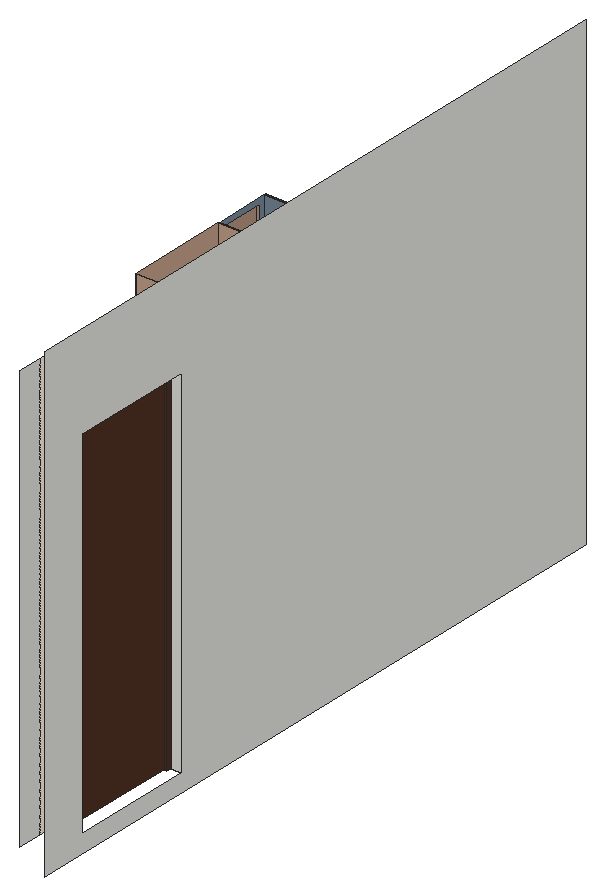
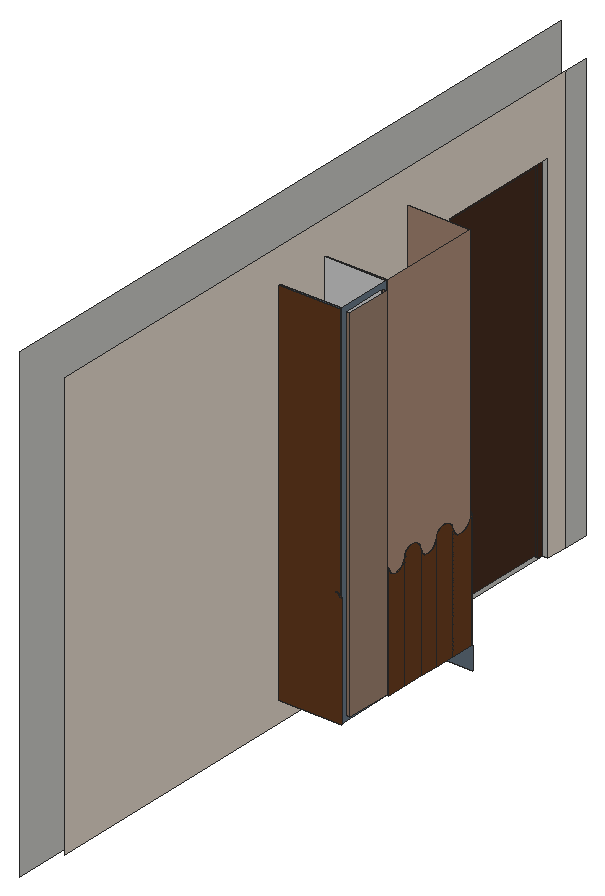
# SketchUp Ruby script. Lengths in inches.
U = 1.inch
M = Sketchup.active_model
def pt(a) = Geom::Point3d.new(a.map { |v| v * U })
def face(e, loops, mat)
  f = e.add_face(loops[0].map { |a| pt(a) })
  loops[1..].each { |l| e.add_face(l.map { |a| pt(a) }).erase! }
  f.material = f.back_material = mat if mat
  f
end
# faces: each face lists its corners as indices into pts; further lists are holes
def faces(e, pts, list, mat = nil) = list.each { |f| face(e, (f[0].is_a?(Array) ? f : [f]).map { |l| l.map { |i| pts[i] } }, mat) }
# xy, xz, yz: faces in a plane at the given z, y or x. An outline is a flat list of corners, or four numbers for a rectangle; further outlines are holes
def ring(l) = l.size == 4 ? [[l[0], l[1]], [l[2], l[1]], [l[2], l[3]], [l[0], l[3]]] : l.each_slice(2).to_a
def flat(e, list, mat, &to3) = list.each { |f| face(e, (f[0].is_a?(Array) ? f : [f]).map { |l| ring(l).map { |u, v| to3.(u, v) } }, mat) }
def xy(e, z, list, mat = nil) = flat(e, list, mat) { |x, y| [x, y, z] }
def xz(e, y, list, mat = nil) = flat(e, list, mat) { |x, z| [x, y, z] }
def yz(e, x, list, mat = nil) = flat(e, list, mat) { |y, z| [x, y, z] }
def lines(e, pts, list) = list.each { |a, b| e.add_line(pt(pts[a]), pt(pts[b])) }
# prism: a flat outline (further loops are holes) pulled along v
def prism(e, loops, v, mat = nil)
  f = face(e, loops, mat); d = Geom::Vector3d.new(v.map { |x| x * U })
  f.pushpull(f.normal.samedirection?(d) ? d.length : -d.length)
end
def box(e, o, s, mat = nil) = prism(e, [[o, [o[0] + s[0], o[1], o[2]], [o[0] + s[0], o[1] + s[1], o[2]], [o[0], o[1] + s[1], o[2]]]], [0, 0, s[2]], mat)
def at(x, y, z, deg = 0) = Geom::Transformation.translation(pt([x, y, z])) * Geom::Transformation.rotation(ORIGIN, Z_AXIS, deg.degrees)
def axes(o, x, y, z) = Geom::Transformation.new([*x, 0, *y, 0, *z, 0, *pt(o).to_a, 1])
def part(name) = M.definitions.add(name)
# library, detail: a bought-in or finely detailed component or shape, given as its bounding box
def library(name, o, s) = part(name).tap { |d| box(d.entities, o, s) }
def detail(e, o, s) = box(e.add_group.entities, o, s)
def put(e, d, t, mat = nil) = e.add_instance(d, t).tap { |i| i.material = mat if mat }
def group(e, t, mat = nil) = e.add_group.tap { |g| g.transformation = t; g.material = mat if mat }.entities
root = M.entities
M.materials.add("Polis06_194").color = [79, 50, 36]
M.materials.add("[0009_Linen]").color = [197, 160, 138]
M.materials.add("[0110_LightSlateGray]1").color = [119, 136, 153]
M.materials.add("[0111_SlateGray]").color = [255, 255, 255]
M.materials.add("[Color D01]").color = [255, 242, 228]
M.materials.add("[Fencing Lattice Natural]").color = [179, 148, 127]
M.materials.add("[Wood Veneer 01]").color = [120, 70, 37]
c1 = part("Flush door")
xy(c1.entities,0,[[0,0,4.72,1.18],[0,34.25,4.72,35.43]],"Polis06_194")
xy(c1.entities,85.26,[[0,1.18,4.72,34.25]],"Polis06_194")
xy(c1.entities,86.61,[[0,0,4.72,35.43]],"Polis06_194")
xz(c1.entities,0,[[0,0,4.72,86.61]],"Polis06_194")
xz(c1.entities,1.18,[[0,0,2.36,85.26],[2.36,0,4.72,85.26]],"Polis06_194")
xz(c1.entities,34.25,[[0,0,4.72,85.26]],"Polis06_194")
xz(c1.entities,35.43,[[0,0,4.72,86.61]],"Polis06_194")
yz(c1.entities,0,[[0,0,1.18,86.61],[34.25,0,35.43,86.61],[1.18,85.26,34.25,86.61]],"Polis06_194")
yz(c1.entities,2.36,[[1.18,0,34.25,0,34.25,85.21,1.18,85.26]],"Polis06_194")
yz(c1.entities,4.72,[[0,0,1.18,86.61],[34.25,0,35.43,86.61],[1.18,85.26,34.25,86.61]],"Polis06_194")
c2 = library("Spot Light\#1",[-5.1,-5.1,-11.05],[10.2,10.2,11.05])
xy(root,13.75,[[535.73,77.57,535.73,78.14,540.39,78.14,539.85,77.57],[539.85,77.57,540.39,78.14,544.32,78.14,543.91,77.57],[543.91,77.57,544.32,78.14,549.07,78.14,548.8,77.57],[548.8,77.57,549.07,78.14,553.89,78.14,553.76,77.57],[553.76,77.57,553.89,78.14,558.07,78.14,558.07,77.57]],"[0009_Linen]")
xy(root,15.58,[[536.14,116.57,553.2,132.48]],"[0110_LightSlateGray]1")
xy(root,15.58,[[534.57,116.57,536.14,132.48]],"[Fencing Lattice Natural]")
xy(root,34.7,[[536.14,116.57,553.2,132.48]],"[0110_LightSlateGray]1")
xy(root,36.7,[[536.14,116.57,553.2,132.48]],"[0110_LightSlateGray]1")
xy(root,55.82,[[536.14,116.57,553.2,132.48]],"[0110_LightSlateGray]1")
xz(root,16.33,[[558.07,6.125,566.72,131.66]])
xz(root,59.9,[[558.07,6.125,566.72,131.66]])
xz(root,77.57,[[535.73,13.75,539.85,13.75,539.85,53.75,539.84,54.31,539.67,54.85,539.34,55.32,538.9,55.6875,538.37,55.92,537.79,56,537.22,55.92,536.6875,55.6875,536.24,55.32,535.92,54.85,535.75,54.31,535.73,53.75],[539.85,13.75,543.91,13.75,543.91,53.75,543.84,53.24,543.64,52.77,543.32,52.36,542.9,52.05,542.41,51.85,541.88,51.78,541.36,51.85,540.87,52.05,540.45,52.36,540.125,52.77,539.92,53.24,539.85,53.75],[543.91,13.75,548.8,13.75,548.8,53.75,548.73,54.375,548.5,54.96,548.11,55.47,547.6,55.86,547,56.1,546.36,56.1875,545.71,56.1,545.11,55.86,544.6,55.47,544.22,54.96,543.98,54.375,543.91,53.75],[548.8,13.75,553.76,13.75,553.76,53.75,553.61,53.18,553.33,52.67,552.93,52.23,552.4375,51.9,551.88,51.7,551.28,51.625,550.68,51.7,550.12,51.9,549.63,52.23,549.23,52.67,548.95,53.18,548.8,53.75],[553.76,13.75,558.07,13.75,558.07,53.75,558.0625,54.34,557.88,54.91,557.55,55.41,557.08,55.8,556.52,56.04,555.92,56.125,555.31,56.04,554.75,55.8,554.29,55.41,553.95,54.91,553.77,54.34,553.76,53.75]],"[Wood Veneer 01]")
xz(root,78.14,[[536.14,13.75,536.14,53.75,535.73,53.75,535.75,54.31,535.92,54.85,536.14,55.16,536.24,55.32,536.6875,55.6875,537.22,55.92,537.79,56,538.37,55.92,538.9,55.6875,539.34,55.32,539.67,54.85,539.84,54.31,539.85,53.75,539.92,53.24,540.125,52.77,540.45,52.36,540.87,52.05,541.36,51.85,541.88,51.78,542.41,51.85,542.9,52.05,543.32,52.36,543.64,52.77,543.84,53.24,543.91,53.75,543.98,54.375,544.22,54.96,544.6,55.47,545.11,55.86,545.71,56.1,546.36,56.1875,547,56.1,547.6,55.86,548.11,55.47,548.5,54.96,548.73,54.375,548.8,53.75,548.95,53.18,549.23,52.67,549.63,52.23,550.12,51.9,550.68,51.7,551.28,51.625,551.88,51.7,552.4375,51.9,552.93,52.23,553.33,52.67,553.61,53.18,553.76,53.75,553.77,54.34,553.95,54.91,554.29,55.41,554.75,55.8,555.31,56.04,555.92,56.125,556.52,56.04,557.08,55.8,557.55,55.41,557.88,54.91,558.0625,54.34,558.07,53.75,558.07,144.125,536.14,144.125,536.14,55.16,536.24,55.32,536.6875,55.6875,537.22,55.92,537.79,56,538.37,55.92,538.9,55.6875,539.34,55.32,539.67,54.85,539.84,54.31,539.85,53.75,539.92,53.24,540.125,52.77,540.45,52.36,540.87,52.05,541.36,51.85,541.88,51.78,542.41,51.85,542.9,52.05,543.32,52.36,543.64,52.77,543.84,53.24,543.91,53.75,543.98,54.375,544.22,54.96,544.6,55.47,545.11,55.86,545.71,56.1,546.36,56.1875,547,56.1,547.6,55.86,548.11,55.47,548.5,54.96,548.73,54.375,548.8,53.75,548.95,53.18,549.23,52.67,549.63,52.23,550.12,51.9,550.68,51.7,551.28,51.625,551.88,51.7,552.4375,51.9,552.93,52.23,553.33,52.67,553.61,53.18,553.76,53.75,553.77,54.34,553.95,54.91,554.29,55.41,554.75,55.8,555.31,56.04,555.92,56.125,556.52,56.04,557.08,55.8,557.55,55.41,557.88,54.91,558.0625,54.34,558.07,53.75,558.07,13.75],[536.14,13.75,558.07,13.75,558.07,53.75,558.0625,54.34,557.88,54.91,557.55,55.41,557.08,55.8,556.52,56.04,555.92,56.125,555.31,56.04,554.75,55.8,554.29,55.41,553.95,54.91,553.77,54.34,553.76,53.75,553.61,53.18,553.33,52.67,552.93,52.23,552.4375,51.9,551.88,51.7,551.28,51.625,550.68,51.7,550.12,51.9,549.63,52.23,549.23,52.67,548.95,53.18,548.8,53.75,548.73,54.375,548.5,54.96,548.11,55.47,547.6,55.86,547,56.1,546.36,56.1875,545.71,56.1,545.11,55.86,544.6,55.47,544.22,54.96,543.98,54.375,543.91,53.75,543.84,53.24,543.64,52.77,543.32,52.36,542.9,52.05,542.41,51.85,541.88,51.78,541.36,51.85,540.87,52.05,540.45,52.36,540.125,52.77,539.92,53.24,539.85,53.75,539.84,54.31,539.67,54.85,539.34,55.32,538.9,55.6875,538.37,55.92,537.79,56,537.22,55.92,536.6875,55.6875,536.24,55.32,536.14,55.16]],"[0009_Linen]")
xz(root,78.14,[[535.07,6.125,558.07,13.75]],"[0110_LightSlateGray]1")
xz(root,78.14,[[535.64,13.75,535.73,53.75],[535.73,13.75,536.14,53.75]],"[Wood Veneer 01]")
xz(root,114.14,[[535.64,13.75,535.64,53.75,536.14,53.75,536.14,144.125,558.07,144.125,558.07,13.75]],"[0009_Linen]")
xz(root,114.74,[[536.14,13.75,558.07,144.125]],"[0111_SlateGray]")
xz(root,116.57,[[536.14,34.7,553.2,36.7],[536.14,55.82,553.2,57.82]])
xz(root,116.57,[[536.14,15.58,553.2,34.7],[536.14,36.7,553.2,55.82]],"[0110_LightSlateGray]1")
xz(root,116.57,[[534.57,15.58,536.14,142.3]],"[Fencing Lattice Natural]")
xz(root,132.48,[[536.14,15.58,553.2,34.7],[536.14,36.7,553.2,55.82]],"[0110_LightSlateGray]1")
xz(root,132.48,[[534.57,15.58,536.14,142.3]],"[Fencing Lattice Natural]")
xz(root,134.3125,[[536.14,13.75,558.07,144.125]],"[0110_LightSlateGray]1")
xz(root,134.91,[[535.64,13.75,558.07,13.75,558.07,144.125,536.14,144.125,536.14,53.75,535.64,53.75]],"[Wood Veneer 01]")
yz(root,534.57,[[116.57,15.58,132.48,142.3]],"[Fencing Lattice Natural]")
yz(root,535.64,[[78.14,13.75,78.14,53.75,78.48,52.93,78.98,52.19,79.64,51.58,80.4,51.13,81.25,50.85,82.14,50.75,83.02,50.85,83.87,51.13,84.64,51.58,85.29,52.19,85.8,52.93,86.14,53.75,86.14,13.75],[86.14,13.75,86.14,53.75,86.36,54.55,86.77,55.28,87.33,55.9,88.03,56.36,88.81,56.65,89.64,56.75,90.47,56.65,91.25,56.36,91.94,55.9,92.51,55.28,92.91,54.55,93.14,53.75,93.14,13.75],[93.14,13.75,93.14,53.75,93.36,52.95,93.77,52.22,94.33,51.6,95.03,51.14,95.81,50.85,96.64,50.75,97.47,50.85,98.25,51.14,98.94,51.6,99.51,52.22,99.91,52.95,100.14,53.75,100.14,13.75],[100.14,13.75,100.14,53.75,100.36,54.55,100.77,55.28,101.33,55.9,102.03,56.36,102.81,56.65,103.64,56.75,104.47,56.65,105.25,56.36,105.94,55.9,106.51,55.28,106.91,54.55,107.14,53.75,107.14,13.75],[107.14,13.75,107.14,53.75,107.36,52.95,107.77,52.22,108.33,51.6,109.03,51.14,109.81,50.85,110.64,50.75,111.47,50.85,112.25,51.14,112.94,51.6,113.51,52.22,113.91,52.95,114.14,53.75,114.14,13.75]],"[Wood Veneer 01]")
yz(root,535.73,[[77.57,13.75,78.14,53.75]],"[Wood Veneer 01]")
yz(root,536.14,[[82.14,50.75,81.25,50.85,80.4,51.13,79.64,51.58,78.98,52.19,78.48,52.93,78.14,53.75,78.14,144.125,114.14,144.125,114.14,53.75,113.91,52.95,113.51,52.22,112.94,51.6,112.25,51.14,111.47,50.85,110.64,50.75,109.81,50.85,109.03,51.14,108.33,51.6,107.77,52.22,107.36,52.95,107.14,53.75,106.91,54.55,106.51,55.28,105.94,55.9,105.25,56.36,104.47,56.65,103.64,56.75,102.81,56.65,102.03,56.36,101.33,55.9,100.77,55.28,100.36,54.55,100.14,53.75,99.91,52.95,99.51,52.22,98.94,51.6,98.25,51.14,97.47,50.85,96.64,50.75,95.81,50.85,95.03,51.14,94.33,51.6,93.77,52.22,93.36,52.95,93.14,53.75,92.91,54.55,92.51,55.28,91.94,55.9,91.25,56.36,90.47,56.65,89.64,56.75,88.81,56.65,88.03,56.36,87.33,55.9,86.77,55.28,86.36,54.55,86.14,53.75,85.8,52.93,85.29,52.19,84.64,51.58,83.87,51.13,83.02,50.85]],"[0009_Linen]")
yz(root,536.14,[[[114.74,13.75,134.3125,144.125],[116.57,15.58,132.48,142.3]],[116.57,34.7,132.48,36.7],[116.57,55.82,132.48,57.82]],"[0110_LightSlateGray]1")
yz(root,553.2,[[116.57,15.58,132.48,34.7],[116.57,36.7,132.48,55.82]],"[0110_LightSlateGray]1")
yz(root,558.07,[[0,6.125,8.65,155.75]])
yz(root,558.07,[[77.57,13.75,78.14,53.75]],"[0009_Linen]")
yz(root,558.07,[[8.65,6.125,8.65,155.75,228.1,155.75,228.1,6.125,59.9,6.125,59.9,131.66,16.33,131.66,16.33,6.125]],"[Color D01]")
yz(root,566.72,[[[0,0,236.75,164.75],[16.33,6.125,59.9,131.66]]])
p = [[536.14,80.4,51.13],[536.14,81.25,50.85],[535.64,81.25,50.85],[535.64,80.4,51.13],[536.14,82.14,50.75],[535.64,82.14,50.75],
  [536.14,83.02,50.85],[535.64,83.02,50.85],[536.14,83.87,51.13],[535.64,83.87,51.13],[536.14,95.03,51.14],[536.14,95.81,50.85],
  [535.64,95.81,50.85],[535.64,95.03,51.14],[536.14,96.64,50.75],[535.64,96.64,50.75],[536.14,97.47,50.85],[535.64,97.47,50.85],
  [536.14,98.25,51.14],[535.64,98.25,51.14],[536.14,109.03,51.14],[536.14,109.81,50.85],[535.64,109.81,50.85],[535.64,109.03,51.14],
  [536.14,110.64,50.75],[535.64,110.64,50.75],[536.14,111.47,50.85],[535.64,111.47,50.85],[536.14,112.25,51.14],[535.64,112.25,51.14],
  [536.14,79.64,51.58],[535.64,79.64,51.58],[536.14,84.64,51.58],[535.64,84.64,51.58],[536.14,94.33,51.6],[535.64,94.33,51.6],
  [536.14,98.94,51.6],[535.64,98.94,51.6],[536.14,108.33,51.6],[535.64,108.33,51.6],[536.14,112.94,51.6],[535.64,112.94,51.6],
  [551.28,78.14,51.625],[550.68,78.14,51.7],[550.68,77.57,51.7],[551.28,77.57,51.625],[551.88,78.14,51.7],[551.88,77.57,51.7],
  [536.14,78.98,52.19],[535.64,78.98,52.19],[536.14,85.29,52.19],[535.64,85.29,52.19],[536.14,93.77,52.22],[535.64,93.77,52.22],
  [536.14,99.51,52.22],[535.64,99.51,52.22],[536.14,107.77,52.22],[535.64,107.77,52.22],[536.14,113.51,52.22],[535.64,113.51,52.22],
  [550.12,78.14,51.9],[550.12,77.57,51.9],[552.4375,78.14,51.9],[552.4375,77.57,51.9],[541.36,78.14,51.85],[540.87,78.14,52.05],
  [540.87,77.57,52.05],[541.36,77.57,51.85],[541.88,78.14,51.78],[541.88,77.57,51.78],[542.41,78.14,51.85],[542.41,77.57,51.85],
  [542.9,78.14,52.05],[542.9,77.57,52.05],[549.63,78.14,52.23],[549.63,77.57,52.23],[552.93,78.14,52.23],[552.93,77.57,52.23],
  [540.45,78.14,52.36],[540.45,77.57,52.36],[543.32,78.14,52.36],[543.32,77.57,52.36],[549.23,78.14,52.67],[549.23,77.57,52.67],
  [553.33,78.14,52.67],[553.33,77.57,52.67],[536.14,78.48,52.93],[535.64,78.48,52.93],[536.14,85.8,52.93],[535.64,85.8,52.93],
  [536.14,93.36,52.95],[535.64,93.36,52.95],[536.14,99.91,52.95],[535.64,99.91,52.95],[536.14,107.36,52.95],[535.64,107.36,52.95],
  [536.14,113.91,52.95],[535.64,113.91,52.95],[540.125,78.14,52.77],[540.125,77.57,52.77],[543.64,78.14,52.77],[543.64,77.57,52.77],
  [548.95,78.14,53.18],[548.95,77.57,53.18],[553.61,78.14,53.18],[553.61,77.57,53.18],[539.92,78.14,53.24],[539.92,77.57,53.24],
  [543.84,78.14,53.24],[543.84,77.57,53.24],[536.14,78.14,53.75],[535.64,78.14,53.75],[535.73,78.14,53.75],[536.14,86.14,53.75],
  [535.64,86.14,53.75],[536.14,93.14,53.75],[535.64,93.14,53.75],[536.14,100.14,53.75],[535.64,100.14,53.75],[536.14,107.14,53.75],
  [535.64,107.14,53.75],[536.14,114.14,53.75],[535.64,114.14,53.75],[539.85,78.14,53.75],[539.85,77.57,53.75],[543.91,78.14,53.75],
  [543.91,77.57,53.75],[548.8,78.14,53.75],[548.8,77.57,53.75],[553.76,78.14,53.75],[553.76,77.57,53.75],[535.75,78.14,54.31],
  [535.73,77.57,53.75],[535.75,77.57,54.31],[539.84,78.14,54.31],[539.84,77.57,54.31],[543.98,78.14,54.375],[543.98,77.57,54.375],
  [548.73,78.14,54.375],[548.73,77.57,54.375],[553.77,78.14,54.34],[553.77,77.57,54.34],[558.07,78.14,53.75],[558.0625,78.14,54.34],
  [558.0625,77.57,54.34],[558.07,77.57,53.75],[536.14,86.36,54.55],[535.64,86.36,54.55],[536.14,92.91,54.55],[535.64,92.91,54.55],
  [536.14,100.36,54.55],[535.64,100.36,54.55],[536.14,106.91,54.55],[535.64,106.91,54.55],[536.14,134.91,53.75],[536.14,135.34,54.59],
  [535.64,135.34,54.59],[535.64,134.91,53.75],[535.92,78.14,54.85],[535.92,77.57,54.85],[539.67,78.14,54.85],[539.67,77.57,54.85],
  [553.95,78.14,54.91],[553.95,77.57,54.91],[557.88,78.14,54.91],[557.88,77.57,54.91],[544.22,78.14,54.96],[544.22,77.57,54.96],
  [548.5,78.14,54.96],[548.5,77.57,54.96],[536.14,86.77,55.28],[535.64,86.77,55.28],[536.14,92.51,55.28],[535.64,92.51,55.28],
  [536.14,100.77,55.28],[535.64,100.77,55.28],[536.14,106.51,55.28],[535.64,106.51,55.28],[536.14,135.92,55.32],[535.64,135.92,55.32],
  [536.14,78.14,55.16],[536.24,77.57,55.32],[536.24,78.14,55.32],[539.34,78.14,55.32],[539.34,77.57,55.32],[554.29,78.14,55.41],
  [554.29,77.57,55.41],[557.55,78.14,55.41],[557.55,77.57,55.41],[544.6,78.14,55.47],[544.6,77.57,55.47],[548.11,78.14,55.47],
  [548.11,77.57,55.47],[536.6875,78.14,55.6875],[536.6875,77.57,55.6875],[538.9,78.14,55.6875],[538.9,77.57,55.6875],[536.14,87.33,55.9],
  [535.64,87.33,55.9],[536.14,91.94,55.9],[535.64,91.94,55.9],[536.14,101.33,55.9],[535.64,101.33,55.9],[536.14,105.94,55.9],
  [535.64,105.94,55.9],[536.14,136.63,55.93],[535.64,136.63,55.93],[554.75,78.14,55.8],[554.75,77.57,55.8],[557.08,78.14,55.8],
  [557.08,77.57,55.8],[545.11,78.14,55.86],[545.11,77.57,55.86],[547.6,78.14,55.86],[547.6,77.57,55.86],[537.22,78.14,55.92],
  [537.22,77.57,55.92],[538.37,78.14,55.92],[538.37,77.57,55.92],[555.31,78.14,56.04],[555.31,77.57,56.04],[556.52,78.14,56.04],
  [556.52,77.57,56.04],[537.79,78.14,56],[537.79,77.57,56],[545.71,78.14,56.1],[545.71,77.57,56.1],[547,78.14,56.1],
  [547,77.57,56.1],[536.14,88.03,56.36],[535.64,88.03,56.36],[536.14,91.25,56.36],[535.64,91.25,56.36],[536.14,102.03,56.36],
  [535.64,102.03,56.36],[536.14,105.25,56.36],[535.64,105.25,56.36],[555.92,78.14,56.125],[555.92,77.57,56.125],[546.36,78.14,56.1875],
  [546.36,77.57,56.1875],[536.14,88.81,56.65],[535.64,88.81,56.65],[536.14,90.47,56.65],[535.64,90.47,56.65],[536.14,102.81,56.65],
  [535.64,102.81,56.65],[536.14,104.47,56.65],[535.64,104.47,56.65],[536.14,89.64,56.75],[535.64,89.64,56.75],[536.14,103.64,56.75],
  [535.64,103.64,56.75]]
faces(root,p,[[0,1,2,3],[1,4,5,2],[4,6,7,5],[6,8,9,7],[10,11,12,13],[11,14,15,12],[14,16,17,15],[16,18,19,17],
  [20,21,22,23],[21,24,25,22],[24,26,27,25],[26,28,29,27],[30,0,3,31],[8,32,33,9],[34,10,13,35],[18,36,37,19],
  [38,20,23,39],[28,40,41,29],[42,43,44,45],[46,42,45,47],[48,30,31,49],[32,50,51,33],[52,34,35,53],[36,54,55,37],
  [56,38,39,57],[40,58,59,41],[43,60,61,44],[62,46,47,63],[64,65,66,67],[68,64,67,69],[70,68,69,71],[72,70,71,73],
  [60,74,75,61],[76,62,63,77],[65,78,79,66],[80,72,73,81],[74,82,83,75],[84,76,77,85],[86,48,49,87],[50,88,89,51],
  [90,52,53,91],[54,92,93,55],[94,56,57,95],[58,96,97,59],[78,98,99,79],[100,80,81,101],[82,102,103,83],[104,84,85,105],
  [98,106,107,99],[108,100,101,109],[110,86,87,111,112],[88,113,114,89],[115,90,91,116],[92,117,118,93],[119,94,95,120],[96,121,122,97],
  [106,123,124,107],[125,108,109,126],[102,127,128,103],[129,104,105,130],[131,112,132,133],[123,134,135,124],[136,125,126,137],[127,138,139,128],
  [140,129,130,141],[142,143,144,145],[113,146,147,114],[148,115,116,149],[117,150,151,118],[152,119,120,153],[154,155,156,157],[158,131,133,159],
  [134,160,161,135],[162,140,141,163],[143,164,165,144],[166,136,137,167],[138,168,169,139],[146,170,171,147],[172,148,149,173],[150,174,175,151],
  [176,152,153,177],[155,178,179,156],[180,158,159,181,182],[160,183,184,161],[185,162,163,186],[164,187,188,165],[189,166,167,190],[168,191,192,169],
  [193,182,181,194],[183,195,196,184],[170,197,198,171],[199,172,173,200],[174,201,202,175],[203,176,177,204],[178,205,206,179],[207,185,186,208],
  [187,209,210,188],[211,189,190,212],[191,213,214,192],[215,193,194,216],[195,217,218,196],[219,207,208,220],[209,221,222,210],[223,215,216,224],
  [217,223,224,218],[225,211,212,226],[213,227,228,214],[197,229,230,198],[231,199,200,232],[201,233,234,202],[235,203,204,236],[237,219,220,238],
  [221,237,238,222],[239,225,226,240],[227,239,240,228],[229,241,242,230],[243,231,232,244],[233,245,246,234],[247,235,236,248],[241,249,250,242],
  [249,243,244,250],[245,251,252,246],[251,247,248,252]],"[Wood Veneer 01]")
put(root,c1,axes([560.43,16.33,6.125],[0.5,0,0],[0,1.22943,0],[0,0,1.44245]))
put(root,c2,at(542.65,124.62,33.82))
put(root,c2,at(542.65,124.62,53.94))
